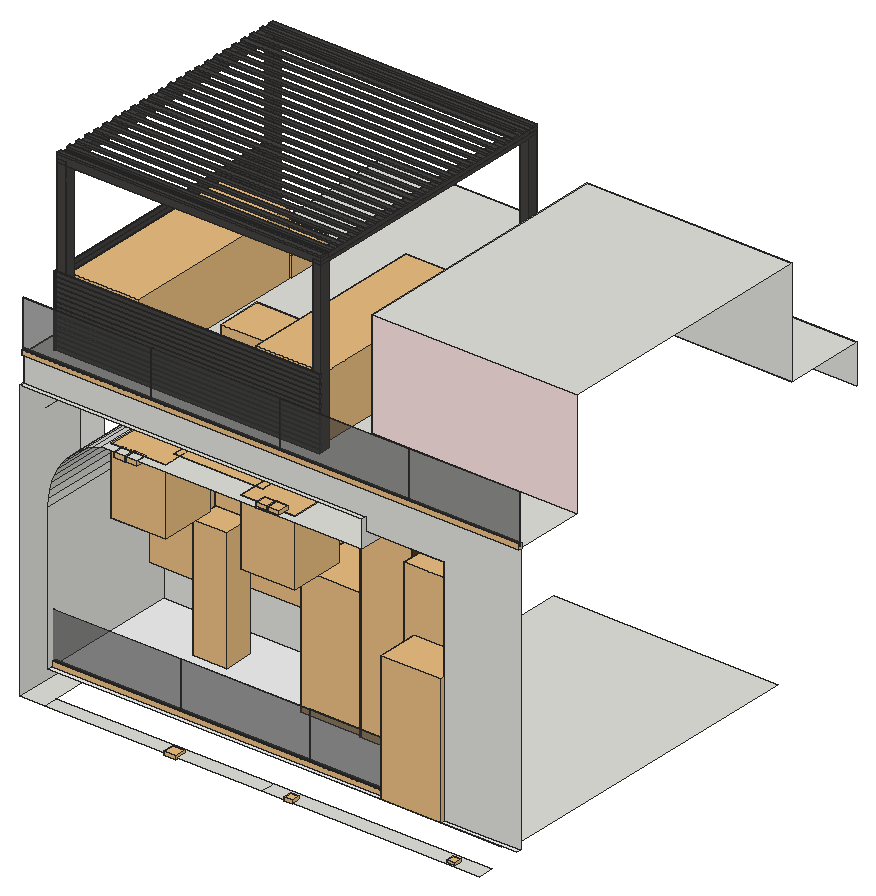
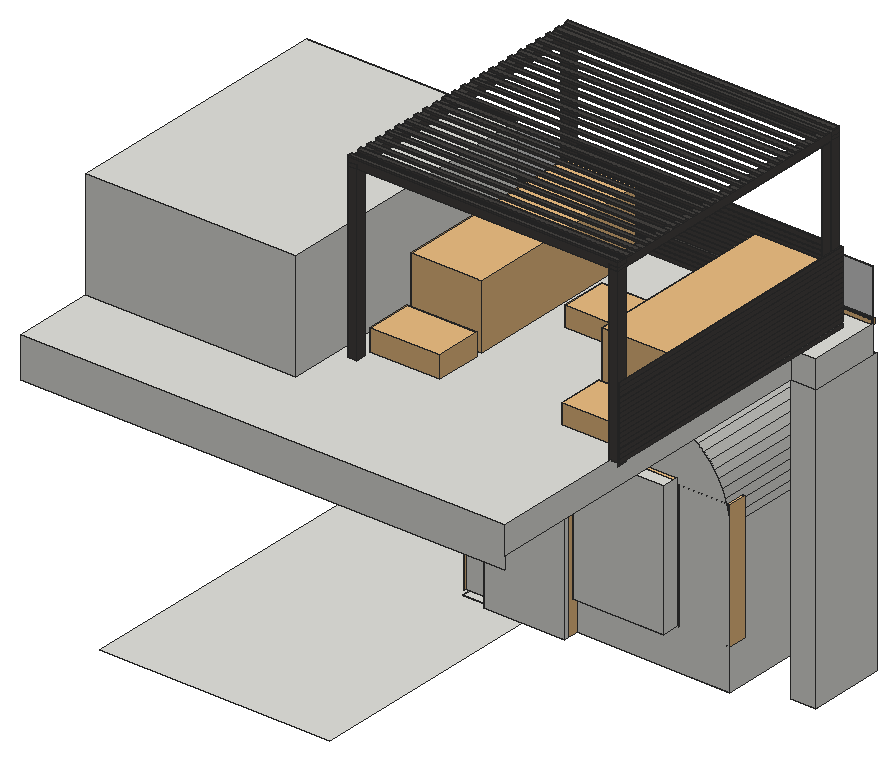
# SketchUp Ruby script. Lengths in inches.
U = 1.inch
M = Sketchup.active_model
def pt(a) = Geom::Point3d.new(a.map { |v| v * U })
def face(e, loops, mat)
  f = e.add_face(loops[0].map { |a| pt(a) })
  loops[1..].each { |l| e.add_face(l.map { |a| pt(a) }).erase! }
  f.material = f.back_material = mat if mat
  f
end
# faces: each face lists its corners as indices into pts; further lists are holes
def faces(e, pts, list, mat = nil) = list.each { |f| face(e, (f[0].is_a?(Array) ? f : [f]).map { |l| l.map { |i| pts[i] } }, mat) }
# xy, xz, yz: faces in a plane at the given z, y or x. An outline is a flat list of corners, or four numbers for a rectangle; further outlines are holes
def ring(l) = l.size == 4 ? [[l[0], l[1]], [l[2], l[1]], [l[2], l[3]], [l[0], l[3]]] : l.each_slice(2).to_a
def flat(e, list, mat, &to3) = list.each { |f| face(e, (f[0].is_a?(Array) ? f : [f]).map { |l| ring(l).map { |u, v| to3.(u, v) } }, mat) }
def xy(e, z, list, mat = nil) = flat(e, list, mat) { |x, y| [x, y, z] }
def xz(e, y, list, mat = nil) = flat(e, list, mat) { |x, z| [x, y, z] }
def yz(e, x, list, mat = nil) = flat(e, list, mat) { |y, z| [x, y, z] }
def lines(e, pts, list) = list.each { |a, b| e.add_line(pt(pts[a]), pt(pts[b])) }
# prism: a flat outline (further loops are holes) pulled along v
def prism(e, loops, v, mat = nil)
  f = face(e, loops, mat); d = Geom::Vector3d.new(v.map { |x| x * U })
  f.pushpull(f.normal.samedirection?(d) ? d.length : -d.length)
end
def box(e, o, s, mat = nil) = prism(e, [[o, [o[0] + s[0], o[1], o[2]], [o[0] + s[0], o[1] + s[1], o[2]], [o[0], o[1] + s[1], o[2]]]], [0, 0, s[2]], mat)
def at(x, y, z, deg = 0) = Geom::Transformation.translation(pt([x, y, z])) * Geom::Transformation.rotation(ORIGIN, Z_AXIS, deg.degrees)
def axes(o, x, y, z) = Geom::Transformation.new([*x, 0, *y, 0, *z, 0, *pt(o).to_a, 1])
def part(name) = M.definitions.add(name)
# library, detail: a bought-in or finely detailed component or shape, given as its bounding box
def library(name, o, s) = part(name).tap { |d| box(d.entities, o, s) }
def detail(e, o, s) = box(e.add_group.entities, o, s)
def put(e, d, t, mat = nil) = e.add_instance(d, t).tap { |i| i.material = mat if mat }
def group(e, t, mat = nil) = e.add_group.tap { |g| g.transformation = t; g.material = mat if mat }.entities
root = M.entities
M.materials.add("Tiles Marble White 03 180cm").color = [241, 241, 241]
M.materials.add("Wood066_2K_Color").color = [89, 51, 19]
M.materials.add("[Color B01]").color = [255, 230, 229]
M.materials.add("[Color M00]").color = [255, 255, 255]
M.materials.add("[Translucent_Glass_Blue]").color = [63, 63, 63]
M.materials["[Translucent_Glass_Blue]"].alpha = 0.35
M.materials.add("[Wood Veneer 01]").color = [68, 66, 64]
M.materials.add("metal railing").color = [165, 165, 165]
M.materials.add("plastic2").color = [86, 86, 86]
c1 = library("Lugstar Premium LED 152 063",[-3.77,-3.75,-3.3125],[7.54,7.53,3.3125])
c2 = part("Tlon Cubo 860 Ceiling 152 005")
xy(c2.entities,-3.04,[[-16.54,-16.54,-16.54,16.54,16.54,-16.54],[16.54,-16.54,-16.54,16.54,16.54,16.54]])
xy(c2.entities,0,[[-16.93,-16.93,16.93,-16.93,-16.93,16.93],[16.93,-16.93,16.93,16.93,-16.93,16.93]])
xz(c2.entities,-16.93,[[-16.93,-3.79,16.93,-3.79,-16.93,0],[16.93,-3.79,16.93,0,-16.93,0]])
xz(c2.entities,-16.3,[[-16.3,-3.66,-16.3,-3.24,16.3,-3.24],[-16.3,-3.66,16.3,-3.24,16.3,-3.66]])
xz(c2.entities,16.3,[[-16.3,-3.66,16.3,-3.24,-16.3,-3.24],[-16.3,-3.66,16.3,-3.66,16.3,-3.24]])
xz(c2.entities,16.93,[[-16.93,-3.79,-16.93,0,16.93,0],[-16.93,-3.79,16.93,0,16.93,-3.79]])
yz(c2.entities,-16.93,[[-16.93,-3.79,-16.93,0,16.93,0],[-16.93,-3.79,16.93,0,16.93,-3.79]])
yz(c2.entities,-16.3,[[-16.3,-3.66,16.3,-3.66,-16.3,-3.24],[16.3,-3.66,16.3,-3.24,-16.3,-3.24]])
yz(c2.entities,16.3,[[-16.3,-3.66,-16.3,-3.24,16.3,-3.66],[16.3,-3.66,-16.3,-3.24,16.3,-3.24]])
yz(c2.entities,16.93,[[-16.93,-3.79,16.93,-3.79,-16.93,0],[16.93,-3.79,16.93,0,-16.93,0]])
p = [[-16.93,-16.93,-3.79],[-16.93,16.93,-3.79],[-16.3,16.3,-3.66],[-16.3,-16.3,-3.66],[16.93,-16.93,-3.79],[16.3,-16.3,-3.66],
  [16.93,16.93,-3.79],[16.3,16.3,-3.66]]
faces(c2.entities,p,[[0,1,2],[2,3,0],[4,0,3],[3,5,4],[6,4,5],[5,7,6],[2,1,6],[6,7,2]])
c3 = library("Planks 104-37 merged",[-27.94,-0.72,0],[55.88,1.44,91.84])
c4 = library("Potted Plant 15",[-14.27,-11.47,0],[24.64,26.73,38.28])
c5 = library("OCDOOR090922",[-8.47,0,0],[8.47,44.51,102.68])
c6 = library("Railing",[0,0,0],[72,2.52,4.03])
c7 = part("railing plastic")
box(c7.entities,[0,0.75,0],[72,0.26,0.68],"plastic2")
box(c7.entities,[0,0,0],[72,0.26,0.68],"plastic2")
c8 = part("Glass Railing pro")
put(c8.entities,c6,axes([0,0,0],[3.06107,0,0],[0,0.7,0],[0,0,0.7]))
put(c8.entities,c7,axes([0,0.53,2.43],[3.06107,0,0],[0,0.7,0],[0,0,0.7]))
c9 = part("sheet glass")
box(c9.entities,[0,0,0],[39.37,0.39,39.37],"[Translucent_Glass_Blue]")
c10 = part("glass stretch")
box(c10.entities,[0,0,0],[39.37,0.39,43.31],"[Translucent_Glass_Blue]")
c11 = part("glass frame")
put(c11.entities,c9,axes([0,0,0],[1.8288,0,0],[0,1.016,0],[0,0,0.7]))
put(c11.entities,c10,axes([216.6,0,0],[0.09644,0,0],[0,1.016,0],[0,0,0.63636]))
put(c11.entities,c9,axes([72.2,0,0],[1.8288,0,0],[0,1.016,0],[0,0,0.7]))
put(c11.entities,c9,axes([144.4,0,0],[1.8288,0,0],[0,1.016,0],[0,0,0.7]))
c12 = part("Glass Railing +")
put(c12.entities,c8,at(0,0,0),"metal railing")
put(c12.entities,c11,at(0,0.74,1.07),"metal railing")
c13 = part("My+Glass_Railing")
put(c13.entities,c12,at(-0.14,0,0))
c14 = library("Jada Standing 001",[-9.65,-9.65,0],[19.3,19.3,65.54])
c15 = library("Window with transom",[0,0,0],[5.2,55.12,70.87])
c16 = library("Plant and PlainPanel 001",[-22.66,-14.09,-22.8],[45.6,14.09,45.6])
c17 = library("Plante \#58",[-0.43,-1.58,0],[20.84,18.06,17.59])
c18 = library("Group\#2",[-0.5,-0.5,-0.1],[129.5625,116.4375,0.2])
c19 = library("Grid Small Coffee Table\#1",[0,0,0],[40.55,19.69,11.8125])
c20 = part("Glass Railing pro\#1")
put(c20.entities,c6,axes([0,0,0],[3.87223,0,0],[0,0.7,0],[0,0,0.7]))
put(c20.entities,c7,axes([0,0.53,2.43],[3.87223,0,0],[0,0.7,0],[0,0,0.7]))
c21 = part("glass frame\#1")
put(c21.entities,c9,axes([0,0,0],[1.8288,0,0],[0,1.016,0],[0,0,0.7]))
put(c21.entities,c10,axes([216.6,0,0],[1.5799,0,0],[0,1.016,0],[0,0,0.63636]))
put(c21.entities,c9,axes([72.2,0,0],[1.8288,0,0],[0,1.016,0],[0,0,0.7]))
put(c21.entities,c9,axes([144.4,0,0],[1.8288,0,0],[0,1.016,0],[0,0,0.7]))
c22 = part("Glass Railing +\#1")
put(c22.entities,c20,at(0,0,0),"metal railing")
put(c22.entities,c21,at(0,0.74,1.07),"metal railing")
c23 = part("My+Glass_Railing\#1")
put(c23.entities,c22,at(-0.18,0,0))
c24 = library("Grid Left/Right End Unit\#1",[0,0,0],[81.54,41,35.59])
c25 = part("Group\#495")
box(c25.entities,[-4,-1,0],[120,1,2])
c26 = part("Group\#494")
xy(c26.entities,0,[[0,0,4,117]])
xy(c26.entities,2,[[0,0,4,4],[0,113,4,117]])
xy(c26.entities,4,[[0,4,4,113]])
xz(c26.entities,0,[[0,0,4,2]])
xz(c26.entities,4,[[0,2,4,4]])
xz(c26.entities,113,[[0,2,4,4]])
xz(c26.entities,117,[[0,0,4,2]])
yz(c26.entities,0,[[0,0,4,2],[4,0,4,4,113,4,113,2,117,2,117,0]])
yz(c26.entities,4,[[0,0,117,0,117,2,113,2,113,4,4,4,4,2,0,2]])
p = [[4,116,4],[0,116,4]]
lines(c26.entities,p,[[0,1]])
xy(root,126.94,[[1630.85,659.65,1644.4,701.28],[1644.4,659.65,1766.5625,667.76],[1766.5625,659.65,1888.73,667.76]])
xy(root,135.03,[[1766.5625,675.17,1766.5625,864.08,1892.58,864.08,1892.58,678.73,1888.73,678.73,1888.73,675.17]])
xy(root,146.4,[[1646.56,659.65,1909.65,659.65,1909.65,661.93,1866.88,661.93,1866.88,694.27,1822.65,694.27,1822.65,697.76,1791.58,697.76,1791.58,740.33,1774.91,740.33,1774.91,748.51,1730.59,748.51,1730.59,740.33,1646.56,740.33]],"Tiles Marble White 03 180cm")
xy(root,168.84,[[1675.43,740.33,1725.05,749.69]])
xy(root,241.6,[[1675.43,740.33,1725.05,749.69]])
xy(root,268.18,[[[1676.34,659.65,1676.34,740.33,1791.58,740.33,1791.58,697.76,1822.65,697.76,1822.65,659.65],[1705.44,674.71,1754.9375,719.15]],[1706.02,675.28,1754.36,718.57]])
xy(root,276.43,[[1822.65,661.93,1866.88,694.27]])
xy(root,283.33,[[1630.85,659.65,1822.65,661.93]])
xy(root,298.4,[[1630.85,661.93,1909.65,661.93,1909.65,701.34,1794.61,701.34,1794.61,852.47,1909.65,852.47,1909.65,897.48,1644.4,897.48,1644.4,701.28,1630.85,701.28]])
xy(root,357.74,[[1794.61,701.34,1909.65,852.47]])
xz(root,661.93,[[1866.88,146.4,1909.65,146.4,1909.65,298.4,1630.85,298.4,1630.85,283.33,1822.65,283.33,1822.65,276.43,1866.88,276.43]])
xz(root,694.27,[[1822.65,146.4,1866.88,276.43]],"Wood066_2K_Color")
xz(root,697.76,[[1791.58,146.4,1822.65,268.18]],"[Color M00]")
xz(root,701.28,[[1630.85,126.94,1644.4,283.33],[1630.85,283.33,1644.4,298.4]])
xz(root,701.34,[[1794.61,298.4,1909.65,357.74]],"[Color B01]")
xz(root,740.33,[[[1646.56,146.4,1730.59,146.4,1730.59,226.54,1731.1875,230.18,1732.25,233.68,1733.74,236.96,1735.64,239.97,1737.9,242.625,1740.47,244.88,1743.31,246.6875,1746.34,248.01,1749.51,248.81,1752.75,249.08,1755.98,248.81,1759.15,248.01,1762.1875,246.6875,1765.02,244.88,1767.6,242.625,1769.85,239.97,1771.75,236.96,1773.25,233.68,1774.31,230.18,1774.91,226.54,1774.91,146.4,1791.58,146.4,1791.58,268.18,1676.34,268.18,1672.13,266.61,1668.12,264.61,1664.34,262.2,1660.83,259.4,1657.64,256.25,1654.8,252.78,1652.34,249.03,1650.29,245.05,1648.67,240.86,1647.5,236.53,1646.79,232.11,1646.56,227.63],[1675.43,168.84,1725.05,241.6]]])
xz(root,748.51,[[1730.59,146.4,1774.91,146.4,1774.91,226.54,1774.31,230.18,1773.25,233.68,1771.75,236.96,1769.85,239.97,1767.6,242.625,1765.02,244.88,1762.1875,246.6875,1759.15,248.01,1755.98,248.81,1752.75,249.08,1749.51,248.81,1746.34,248.01,1743.31,246.6875,1740.47,244.88,1737.9,242.625,1735.64,239.97,1733.74,236.96,1732.25,233.68,1731.1875,230.18,1730.59,226.54]])
xz(root,749.69,[[1675.43,168.84,1725.05,241.6]])
xz(root,852.47,[[1794.61,298.4,1909.65,357.74]])
xz(root,897.48,[[1644.4,276.43,1909.65,298.4]])
yz(root,1630.85,[[659.65,126.94,701.28,283.33],[661.93,283.33,701.28,298.4]])
yz(root,1640.19,[[819.61,296.4,824.77,392.37]],"[Wood Veneer 01]")
yz(root,1644.4,[[701.28,283.33,897.48,298.4]])
yz(root,1646.56,[[659.65,146.4,740.33,227.63]])
yz(root,1675.43,[[740.33,168.84,749.69,241.6]])
yz(root,1725.05,[[740.33,168.84,749.69,241.6]])
yz(root,1730.59,[[740.33,146.4,748.51,226.54]])
yz(root,1774.91,[[740.33,146.4,748.51,226.54]])
yz(root,1791.58,[[697.76,146.4,740.33,268.18]],"[Color M00]")
yz(root,1794.61,[[701.34,298.4,852.47,357.74]])
yz(root,1822.65,[[659.65,268.18,694.27,268.18,694.27,276.43,661.93,276.43,661.93,283.33,659.65,283.33]])
yz(root,1822.65,[[694.27,146.4,697.76,268.18]],"Wood066_2K_Color")
yz(root,1866.88,[[661.93,146.4,694.27,276.43]])
p = [[1731.1875,740.33,230.18],[1730.59,740.33,226.54],[1730.59,748.51,226.54],[1731.1875,748.51,230.18],[1774.91,740.33,226.54],[1774.31,740.33,230.18],
  [1774.31,748.51,230.18],[1774.91,748.51,226.54],[1646.79,740.33,232.11],[1646.79,659.65,232.11],[1646.56,659.65,227.63],[1646.56,740.33,227.63],
  [1732.25,740.33,233.68],[1732.25,748.51,233.68],[1773.25,740.33,233.68],[1773.25,748.51,233.68],[1647.5,740.33,236.53],[1647.5,659.65,236.53],
  [1733.74,740.33,236.96],[1733.74,748.51,236.96],[1771.75,740.33,236.96],[1771.75,748.51,236.96],[1648.67,740.33,240.86],[1648.67,659.65,240.86],
  [1735.64,740.33,239.97],[1735.64,748.51,239.97],[1769.85,740.33,239.97],[1769.85,748.51,239.97],[1737.9,740.33,242.625],[1737.9,748.51,242.625],
  [1767.6,740.33,242.625],[1767.6,748.51,242.625],[1650.29,740.33,245.05],[1650.29,659.65,245.05],[1740.47,740.33,244.88],[1740.47,748.51,244.88],
  [1765.02,740.33,244.88],[1765.02,748.51,244.88],[1743.31,740.33,246.6875],[1743.31,748.51,246.6875],[1762.1875,740.33,246.6875],[1762.1875,748.51,246.6875],
  [1652.34,740.33,249.03],[1652.34,659.65,249.03],[1746.34,740.33,248.01],[1746.34,748.51,248.01],[1759.15,740.33,248.01],[1759.15,748.51,248.01],
  [1749.51,740.33,248.81],[1749.51,748.51,248.81],[1755.98,740.33,248.81],[1755.98,748.51,248.81],[1752.75,740.33,249.08],[1752.75,748.51,249.08],
  [1654.8,740.33,252.78],[1654.8,659.65,252.78],[1657.64,740.33,256.25],[1657.64,659.65,256.25],[1660.83,740.33,259.4],[1660.83,659.65,259.4],
  [1664.34,740.33,262.2],[1664.34,659.65,262.2],[1668.12,740.33,264.61],[1668.12,659.65,264.61],[1672.13,740.33,266.61],[1672.13,659.65,266.61],
  [1676.34,740.33,268.18],[1676.34,659.65,268.18],[1644.4,660.2,276.43],[1644.4,701.28,276.43],[1788.3,824.77,298.37],[1788.3,824.77,394.37],
  [1640.19,679,296.4],[1640.19,679,392.37],[1640.19,819.61,392.37],[1645.13,673.84,386.71],[1645.13,673.84,392.37],[1645.13,673.84,296.4],
  [1645.13,679,296.4],[1645.13,673.84,300.37],[1645.13,673.84,383.88],[1788.3,679,394.37]]
faces(root,p,[[0,1,2,3],[4,5,6,7],[8,9,10,11],[12,0,3,13],[5,14,15,6],[16,17,9,8],[18,12,13,19],[14,20,21,15],
  [22,23,17,16],[24,18,19,25],[20,26,27,21],[28,24,25,29],[26,30,31,27],[32,33,23,22],[34,28,29,35],[30,36,37,31],
  [38,34,35,39],[36,40,41,37],[42,43,33,32],[44,38,39,45],[40,46,47,41],[48,44,45,49],[46,50,51,47],[52,48,49,53],
  [50,52,53,51],[54,55,43,42],[56,57,55,54],[58,59,57,56],[60,61,59,58],[62,63,61,60],[64,65,63,62],[66,67,65,64]])
lines(root,p,[[68,69],[70,71],[72,73],[73,74],[75,76],[77,78],[78,72],[79,80],[81,71]])
put(root,c1,axes([1715.17,662.25,128.07],[0.86778,0,0],[0,0.81438,0],[0,0,0.66752]))
put(root,c1,axes([1871.6,662.82,128],[0.60684,0,0],[0,0.60684,0],[0,0,0.60684]))
put(root,c1,axes([1781.2,661.92,128.21],[0.60684,0,0],[0,0.60684,0],[0,0,0.60684]))
put(root,c2,axes([1793.2,721.1875,135.03],[0.5,0,0],[0,0.5,0],[0,0,0.5]))
put(root,c3,axes([1791.36,719.25,146.37],[0,0.78784,0],[-0.4697,0,0],[0,0,1.32586]))
put(root,c4,axes([1776.72,713.05,146.39],[1.37999,0,0],[0,1.27982,0],[0,0,1.8788]))
put(root,c3,axes([1806.76,697.42,146.4],[0.54334,0,0],[0,0.4697,0],[0,0,1.32586]))
put(root,c5,at(1774.91,745.7,146.4,90))
put(root,c4,axes([1852.58,674.33,146.4],[1.37999,0,0],[0,1.27982,0],[0,0,1.8788]))
put(root,c13,at(1646.63,661.93,146.4))
put(root,c14,axes([1698.04,716.67,146.4],[1,0,0],[0,0.85,0],[0,0,1.0368]))
put(root,c15,axes([1725.09,740.3125,168.82],[0,0.385,0],[-0.9009,0,0],[0,0,1.02701]))
put(root,c16,axes([1660.55,740.33,203.74],[0.61749,0,0],[0,0.71995,0],[0,0,1.53076]))
put(root,c16,axes([1844.02,694.27,218.27],[0.74324,0,0],[0,0.77,0],[0,0,1.52075]))
put(root,c17,axes([1751.35,666.96,230.92],[1.4573,0,0],[0,1.70958,0],[0,0,2.11841]))
put(root,c17,axes([1678.37,667.54,230.92],[1.4573,0,0],[0,1.70958,0],[0,0,2.11841]))
put(root,c1,axes([1693.15,662.7,268.18],[0.81428,0,0],[0,0.81428,0],[0,0,0.81428]))
put(root,c1,axes([1686.625,662.7,268.18],[0.81428,0,0],[0,0.81428,0],[0,0,0.81428]))
put(root,c1,axes([1765.2,713.68,268.8125],[0.81428,0,0],[0,0.81428,0],[0,0,0.81428]))
put(root,c1,axes([1771.72,713.68,268.8125],[0.81428,0,0],[0,0.81428,0],[0,0,0.81428]))
put(root,c1,axes([1689.43,713.68,268.8125],[0.81428,0,0],[0,0.81428,0],[0,0,0.81428]))
put(root,c1,axes([1682.91,713.68,268.8125],[0.81428,0,0],[0,0.81428,0],[0,0,0.81428]))
put(root,c2,axes([1729.93,693.26,268.18],[0.5,0,0],[0,0.5,0],[0,0,0.5]))
put(root,c1,axes([1771.77,663.92,270.09],[0.81428,0,0],[0,0.81428,0],[0,0,0.81428]))
put(root,c1,axes([1765.25,663.92,270.09],[0.81428,0,0],[0,0.81428,0],[0,0,0.81428]))
put(root,c18,axes([1705.44,674.71,268.18],[0.385,0,0],[0,0.385,0],[0,0,0.385]))
put(root,c1,axes([1845.89,675.3125,276.43],[0.81428,0,0],[0,0.81428,0],[0,0,0.81428]))
put(root,c1,axes([1839.37,675.3125,276.43],[0.81428,0,0],[0,0.81428,0],[0,0,0.81428]))
put(root,c19,axes([1642.18,788.15,297.18],[0.9405,0,0],[0,1.29,0],[0,0,1]))
put(root,c19,axes([1694.07,721.01,297.22],[0.9405,0,0],[0,1.29,0],[0,0,1]))
put(root,c23,at(1631.03,660.76,297.86))
g1 = group(root,at(1640.19,673.84,298.37),"[Wood Veneer 01]")
box(g1,[0,0,0],[4.9375,5.16,94])
g2 = group(root,at(1783.37,673.84,298.37),"[Wood Veneer 01]")
box(g2,[0,0,0],[4.9375,5.16,94])
g3 = group(root,at(1783.37,819.61,298.37),"[Wood Veneer 01]")
box(g3,[0,0,0],[4.9375,5.16,94])
g4 = group(root,at(1640.19,819.61,298.37),"[Wood Veneer 01]")
xy(g4,94,[[0,0,4.9375,5.16]])
xz(g4,5.16,[[0,0,4.9375,94]])
yz(g4,4.9375,[[0,0,5.16,94]])
p = [[4.9375,0,0],[0,0,0]]
lines(g4,p,[[0,1]])
put(root,c24,axes([1784.24,681.27,298.4],[0,1.29,0],[-0.9405,0,0],[0,0,1]))
put(root,c24,axes([1641.37,681.27,298.4],[0,1.29,0],[0.9405,0,0],[0,0,1]))
put(root,c19,axes([1745.52,790,298.4],[0.9405,0,0],[0,1.29,0],[0,0,1]))
put(root,c25,axes([1645.13,673.84,298.4],[1.23425,0,0],[0,1.29,0],[0,0,1]),"[Wood Veneer 01]")
put(root,c25,axes([1640.02,819.69,298.4],[0,-1.2685,0],[0.9405,0,0],[0,0,1]),"[Wood Veneer 01]")
put(root,c25,axes([1640.02,819.69,300.96],[0,-1.2685,0],[0.9405,0,0],[0,0,1]),"[Wood Veneer 01]")
put(root,c25,axes([1645.14,673.84,300.96],[1.23425,0,0],[0,1.29,0],[0,0,1]),"[Wood Veneer 01]")
put(root,c25,axes([1645.13,673.84,303.4],[1.23425,0,0],[0,1.29,0],[0,0,1]),"[Wood Veneer 01]")
put(root,c25,axes([1640.02,819.69,303.4],[0,-1.2685,0],[0.9405,0,0],[0,0,1]),"[Wood Veneer 01]")
put(root,c25,axes([1640.02,819.69,305.96],[0,-1.2685,0],[0.9405,0,0],[0,0,1]),"[Wood Veneer 01]")
put(root,c25,axes([1645.14,673.84,305.96],[1.23425,0,0],[0,1.29,0],[0,0,1]),"[Wood Veneer 01]")
put(root,c25,axes([1645.13,673.84,308.4],[1.23425,0,0],[0,1.29,0],[0,0,1]),"[Wood Veneer 01]")
put(root,c25,axes([1640.02,819.69,308.4],[0,-1.2685,0],[0.9405,0,0],[0,0,1]),"[Wood Veneer 01]")
put(root,c25,axes([1640.02,819.69,310.96],[0,-1.2685,0],[0.9405,0,0],[0,0,1]),"[Wood Veneer 01]")
put(root,c25,axes([1645.14,673.84,310.96],[1.23425,0,0],[0,1.29,0],[0,0,1]),"[Wood Veneer 01]")
put(root,c25,axes([1645.13,673.84,313.4],[1.23425,0,0],[0,1.29,0],[0,0,1]),"[Wood Veneer 01]")
put(root,c25,axes([1640.02,819.69,313.4],[0,-1.2685,0],[0.9405,0,0],[0,0,1]),"[Wood Veneer 01]")
put(root,c25,axes([1640.02,819.69,315.96],[0,-1.2685,0],[0.9405,0,0],[0,0,1]),"[Wood Veneer 01]")
put(root,c25,axes([1645.14,673.84,315.96],[1.23425,0,0],[0,1.29,0],[0,0,1]),"[Wood Veneer 01]")
put(root,c25,axes([1645.13,673.84,318.4],[1.23425,0,0],[0,1.29,0],[0,0,1]),"[Wood Veneer 01]")
put(root,c25,axes([1640.02,819.69,318.4],[0,-1.2685,0],[0.9405,0,0],[0,0,1]),"[Wood Veneer 01]")
put(root,c25,axes([1640.02,819.69,320.96],[0,-1.2685,0],[0.9405,0,0],[0,0,1]),"[Wood Veneer 01]")
put(root,c25,axes([1645.14,673.84,320.96],[1.23425,0,0],[0,1.29,0],[0,0,1]),"[Wood Veneer 01]")
put(root,c25,axes([1645.13,673.84,323.4],[1.23425,0,0],[0,1.29,0],[0,0,1]),"[Wood Veneer 01]")
put(root,c25,axes([1640.02,819.69,323.4],[0,-1.2685,0],[0.9405,0,0],[0,0,1]),"[Wood Veneer 01]")
put(root,c25,axes([1640.02,819.69,325.96],[0,-1.2685,0],[0.9405,0,0],[0,0,1]),"[Wood Veneer 01]")
put(root,c25,axes([1645.14,673.84,325.96],[1.23425,0,0],[0,1.29,0],[0,0,1]),"[Wood Veneer 01]")
put(root,c25,axes([1645.13,673.84,328.4],[1.23425,0,0],[0,1.29,0],[0,0,1]),"[Wood Veneer 01]")
put(root,c25,axes([1640.02,819.69,328.4],[0,-1.2685,0],[0.9405,0,0],[0,0,1]),"[Wood Veneer 01]")
put(root,c25,axes([1640.02,819.69,330.96],[0,-1.2685,0],[0.9405,0,0],[0,0,1]),"[Wood Veneer 01]")
put(root,c25,axes([1645.14,673.84,330.96],[1.23425,0,0],[0,1.29,0],[0,0,1]),"[Wood Veneer 01]")
put(root,c25,axes([1645.13,673.84,333.4],[1.23425,0,0],[0,1.29,0],[0,0,1]),"[Wood Veneer 01]")
put(root,c25,axes([1640.02,819.69,333.4],[0,-1.2685,0],[0.9405,0,0],[0,0,1]),"[Wood Veneer 01]")
put(root,c25,axes([1640.02,819.69,335.96],[0,-1.2685,0],[0.9405,0,0],[0,0,1]),"[Wood Veneer 01]")
put(root,c25,axes([1645.14,673.84,335.96],[1.23425,0,0],[0,1.29,0],[0,0,1]),"[Wood Veneer 01]")
g5 = group(root,at(1640.19,673.84,394.37),"[Wood Veneer 01]")
prism(g5,[[[0,0,2],[0,0,0],[4.9375,0,0],[4.9375,0,-2],[143.17,0,-2],[143.17,0,0],[148.11,0,0],[148.11,0,2]]],[0,5.16,0])
g6 = group(root,at(1640.19,819.61,394.37),"[Wood Veneer 01]")
prism(g6,[[[0,0,2],[0,0,0],[4.9375,0,0],[4.9375,0,-2],[143.17,0,-2],[143.17,0,0],[148.11,0,0],[148.11,0,2]]],[0,5.16,0])
put(root,c26,axes([1640.19,673.84,392.37],[1.23425,0,0],[0,1.29,0],[0,0,1]),"[Wood Veneer 01]")
put(root,c26,axes([1783.37,673.84,392.37],[1.23425,0,0],[0,1.29,0],[0,0,1]),"[Wood Veneer 01]")
put(root,c25,axes([1645.13,673.84,396.37],[1.23425,0,0],[0,0,-1],[0,1.29,0]),"[Wood Veneer 01]")
put(root,c25,axes([1645.13,680.29,396.37],[1.23425,0,0],[0,0,-1],[0,1.29,0]),"[Wood Veneer 01]")
put(root,c25,axes([1645.13,686.74,396.37],[1.23425,0,0],[0,0,-1],[0,1.29,0]),"[Wood Veneer 01]")
put(root,c25,axes([1645.13,699.64,396.37],[1.23425,0,0],[0,0,-1],[0,1.29,0]),"[Wood Veneer 01]")
put(root,c25,axes([1645.13,693.19,396.37],[1.23425,0,0],[0,0,-1],[0,1.29,0]),"[Wood Veneer 01]")
put(root,c25,axes([1645.13,712.54,396.37],[1.23425,0,0],[0,0,-1],[0,1.29,0]),"[Wood Veneer 01]")
put(root,c25,axes([1645.13,706.09,396.37],[1.23425,0,0],[0,0,-1],[0,1.29,0]),"[Wood Veneer 01]")
put(root,c25,axes([1645.13,744.79,396.37],[1.23425,0,0],[0,0,-1],[0,1.29,0]),"[Wood Veneer 01]")
put(root,c25,axes([1645.13,731.89,396.37],[1.23425,0,0],[0,0,-1],[0,1.29,0]),"[Wood Veneer 01]")
put(root,c25,axes([1645.13,718.99,396.37],[1.23425,0,0],[0,0,-1],[0,1.29,0]),"[Wood Veneer 01]")
put(root,c25,axes([1645.13,725.44,396.37],[1.23425,0,0],[0,0,-1],[0,1.29,0]),"[Wood Veneer 01]")
put(root,c25,axes([1645.13,738.34,396.37],[1.23425,0,0],[0,0,-1],[0,1.29,0]),"[Wood Veneer 01]")
put(root,c25,axes([1645.13,789.94,396.37],[1.23425,0,0],[0,0,-1],[0,1.29,0]),"[Wood Veneer 01]")
put(root,c25,axes([1645.13,764.14,396.37],[1.23425,0,0],[0,0,-1],[0,1.29,0]),"[Wood Veneer 01]")
put(root,c25,axes([1645.13,770.59,396.37],[1.23425,0,0],[0,0,-1],[0,1.29,0]),"[Wood Veneer 01]")
put(root,c25,axes([1645.13,796.39,396.37],[1.23425,0,0],[0,0,-1],[0,1.29,0]),"[Wood Veneer 01]")
put(root,c25,axes([1645.13,757.69,396.37],[1.23425,0,0],[0,0,-1],[0,1.29,0]),"[Wood Veneer 01]")
put(root,c25,axes([1645.13,777.04,396.37],[1.23425,0,0],[0,0,-1],[0,1.29,0]),"[Wood Veneer 01]")
put(root,c25,axes([1645.13,802.84,396.37],[1.23425,0,0],[0,0,-1],[0,1.29,0]),"[Wood Veneer 01]")
put(root,c25,axes([1645.13,783.49,396.37],[1.23425,0,0],[0,0,-1],[0,1.29,0]),"[Wood Veneer 01]")
put(root,c25,axes([1645.13,809.29,396.37],[1.23425,0,0],[0,0,-1],[0,1.29,0]),"[Wood Veneer 01]")
put(root,c25,axes([1645.13,751.24,396.37],[1.23425,0,0],[0,0,-1],[0,1.29,0]),"[Wood Veneer 01]")
put(root,c25,axes([1645.13,822.19,396.37],[1.23425,0,0],[0,0,-1],[0,1.29,0]),"[Wood Veneer 01]")
put(root,c25,axes([1645.13,815.74,396.37],[1.23425,0,0],[0,0,-1],[0,1.29,0]),"[Wood Veneer 01]")
